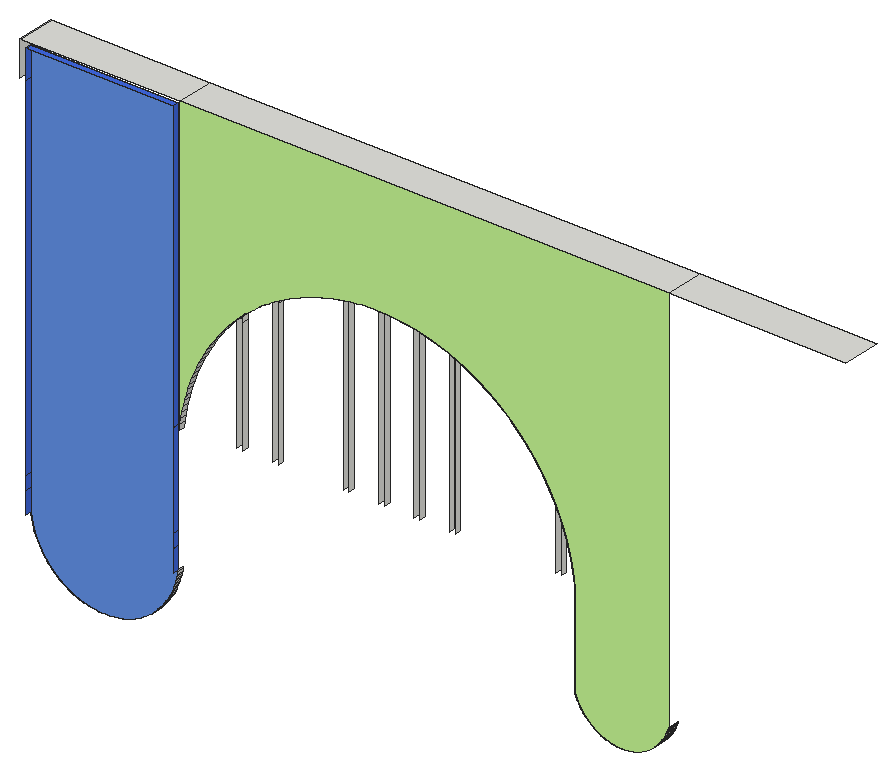
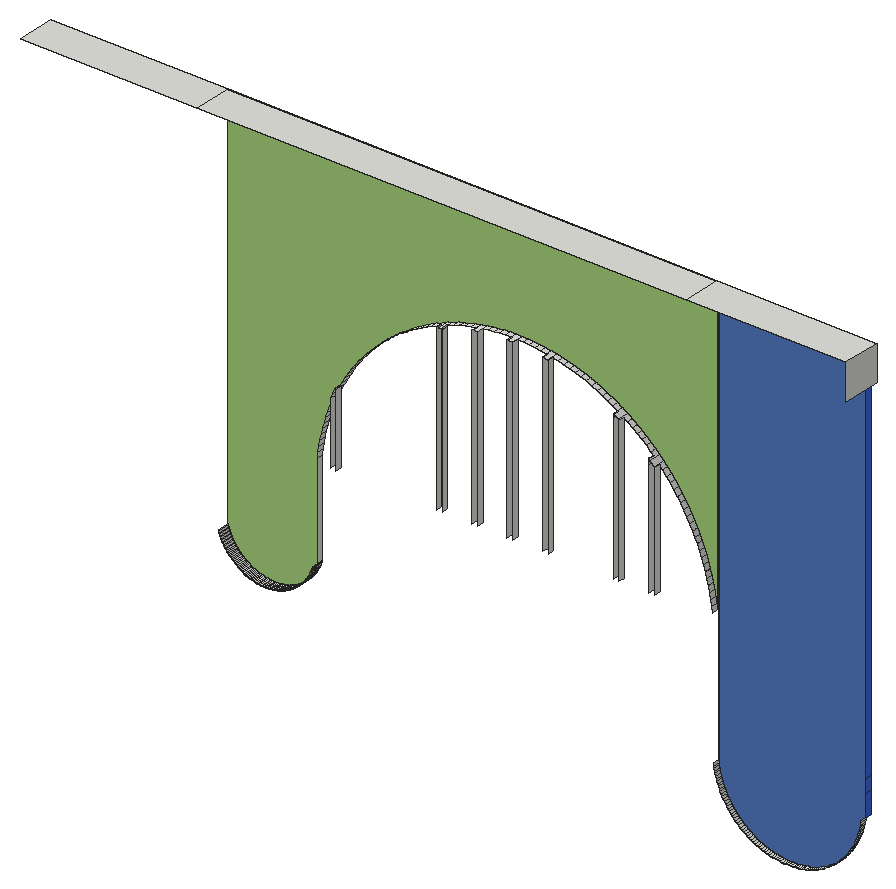
# SketchUp Ruby script. Lengths in inches.
U = 1.inch
M = Sketchup.active_model
def pt(a) = Geom::Point3d.new(a.map { |v| v * U })
def face(e, loops, mat)
  f = e.add_face(loops[0].map { |a| pt(a) })
  loops[1..].each { |l| e.add_face(l.map { |a| pt(a) }).erase! }
  f.material = f.back_material = mat if mat
  f
end
# faces: each face lists its corners as indices into pts; further lists are holes
def faces(e, pts, list, mat = nil) = list.each { |f| face(e, (f[0].is_a?(Array) ? f : [f]).map { |l| l.map { |i| pts[i] } }, mat) }
# xy, xz, yz: faces in a plane at the given z, y or x. An outline is a flat list of corners, or four numbers for a rectangle; further outlines are holes
def ring(l) = l.size == 4 ? [[l[0], l[1]], [l[2], l[1]], [l[2], l[3]], [l[0], l[3]]] : l.each_slice(2).to_a
def flat(e, list, mat, &to3) = list.each { |f| face(e, (f[0].is_a?(Array) ? f : [f]).map { |l| ring(l).map { |u, v| to3.(u, v) } }, mat) }
def xy(e, z, list, mat = nil) = flat(e, list, mat) { |x, y| [x, y, z] }
def xz(e, y, list, mat = nil) = flat(e, list, mat) { |x, z| [x, y, z] }
def yz(e, x, list, mat = nil) = flat(e, list, mat) { |y, z| [x, y, z] }
def lines(e, pts, list) = list.each { |a, b| e.add_line(pt(pts[a]), pt(pts[b])) }
# prism: a flat outline (further loops are holes) pulled along v
def prism(e, loops, v, mat = nil)
  f = face(e, loops, mat); d = Geom::Vector3d.new(v.map { |x| x * U })
  f.pushpull(f.normal.samedirection?(d) ? d.length : -d.length)
end
def box(e, o, s, mat = nil) = prism(e, [[o, [o[0] + s[0], o[1], o[2]], [o[0] + s[0], o[1] + s[1], o[2]], [o[0], o[1] + s[1], o[2]]]], [0, 0, s[2]], mat)
def at(x, y, z, deg = 0) = Geom::Transformation.translation(pt([x, y, z])) * Geom::Transformation.rotation(ORIGIN, Z_AXIS, deg.degrees)
def axes(o, x, y, z) = Geom::Transformation.new([*x, 0, *y, 0, *z, 0, *pt(o).to_a, 1])
def part(name) = M.definitions.add(name)
# library, detail: a bought-in or finely detailed component or shape, given as its bounding box
def library(name, o, s) = part(name).tap { |d| box(d.entities, o, s) }
def detail(e, o, s) = box(e.add_group.entities, o, s)
def put(e, d, t, mat = nil) = e.add_instance(d, t).tap { |i| i.material = mat if mat }
def group(e, t, mat = nil) = e.add_group.tap { |g| g.transformation = t; g.material = mat if mat }.entities
root = M.entities
M.materials.add("[0101_CornflowerBlue]").color = [100, 149, 237]
M.materials.add("[0102_RoyalBlue]").color = [65, 105, 225]
M.materials.add("[Color F02]").color = [204, 255, 153]
xy(root,18.939,[[13.316,5.25,13.684,6.25]])
xy(root,30.001,[[101.892,4.25,102.108,6.25]])
xy(root,81.996,[[60.003,4.25,60.997,6.25]])
xy(root,101,[[1,4.25,26,5.25]],"[0102_RoyalBlue]")
xy(root,102,[[0,4.25,27,10.75],[27,4.25,110,10.75],[110,4.25,140,10.75]])
xz(root,4.25,[[101.892,30.001,102.108,30.001,102.325,30.006,102.541,30.018,102.757,30.034,102.973,30.057,103.1875,30.085,103.402,30.119,103.615,30.158,103.827,30.203,104.037,30.253,104.247,30.309,104.455,30.37,104.661,30.436,104.865,30.508,105.068,30.585,105.268,30.668,105.466,30.755,105.662,30.848,105.856,30.946,106.046,31.048,106.234,31.156,106.419,31.268,106.602,31.386,106.781,31.508,106.957,31.634,107.129,31.765,107.298,31.901,107.463,32.041,107.625,32.185,107.783,32.333,107.937,32.486,108.087,32.642,108.233,32.802,108.375,32.966,108.512,33.134,108.645,33.305,108.774,33.479,108.898,33.657,109.017,33.838,109.131,34.022,109.241,34.209,109.346,34.398,109.446,34.591,109.54,34.785,109.63,34.983,109.715,35.182,109.794,35.384,109.868,35.587,109.937,35.793,110,36,110,102,27,102,27,52,27.124,52.987,27.277,53.969,27.459,54.947,27.669,55.919,27.909,56.885,28.162,57.792,28.176,57.842,28.472,58.792,28.795,59.732,29.147,60.663,29.525,61.582,29.931,62.491,30.363,63.386,30.821,64.269,31.305,65.138,31.815,65.992,32.35,66.83,32.909,67.653,33.492,68.458,34.098,69.246,34.728,70.016,35.38,70.767,36.054,71.499,36.749,72.21,37.465,72.9,38.201,73.569,38.956,74.216,39.731,74.84,40.523,75.441,41.332,76.019,42.159,76.572,43.001,77.101,43.859,77.605,44.73,78.083,45.616,78.536,46.515,78.962,47.426,79.361,48.348,79.733,49.281,80.078,50.223,80.395,51.175,80.684,52.135,80.945,53.102,81.178,54.075,81.382,55.054,81.557,56.038,81.703,57.025,81.82,58.016,81.908,59.009,81.967,60.003,81.996,60.997,81.996,61.991,81.967,62.984,81.908,63.975,81.82,64.962,81.703,65.946,81.557,66.925,81.382,67.898,81.178,68.865,80.945,69.825,80.684,70.777,80.395,71.719,80.078,72.652,79.733,73.574,79.361,74.485,78.962,75.384,78.536,76.27,78.083,77.141,77.605,77.999,77.101,78.841,76.572,79.668,76.019,80.477,75.441,81.269,74.84,82.044,74.216,82.799,73.569,83.535,72.9,84.251,72.21,84.946,71.499,85.62,70.767,86.272,70.016,86.902,69.246,87.508,68.458,88.091,67.653,88.65,66.83,89.185,65.992,89.695,65.138,90.179,64.269,90.637,63.386,91.069,62.491,91.475,61.582,91.853,60.663,92.205,59.732,92.528,58.792,92.824,57.842,93.091,56.885,93.331,55.919,93.541,54.947,93.723,53.969,93.876,52.987,94,52,94,36,94.063,35.793,94.132,35.587,94.206,35.384,94.285,35.182,94.37,34.983,94.46,34.785,94.554,34.591,94.654,34.398,94.759,34.209,94.869,34.022,94.983,33.838,95.102,33.657,95.226,33.479,95.355,33.305,95.488,33.134,95.625,32.966,95.767,32.802,95.913,32.642,96.063,32.486,96.217,32.333,96.375,32.185,96.537,32.041,96.702,31.901,96.871,31.765,97.043,31.634,97.219,31.508,97.398,31.386,97.581,31.268,97.766,31.156,97.954,31.048,98.144,30.946,98.338,30.848,98.534,30.755,98.732,30.668,98.932,30.585,99.135,30.508,99.339,30.436,99.545,30.37,99.753,30.309,99.963,30.253,100.173,30.203,100.385,30.158,100.598,30.119,100.8125,30.085,101.027,30.057,101.243,30.034,101.459,30.018,101.675,30.006]],"[Color F02]")
xz(root,5.25,[[13.316,18.939,13.684,18.939,14.053,18.95,14.421,18.971,14.788,19.004,15.154,19.047,15.519,19.1,15.882,19.165,16.243,19.24,16.601,19.325,16.957,19.421,17.31,19.528,17.66,19.644,18.006,19.771,18.348,19.908,18.686,20.055,19.02,20.212,19.349,20.378,19.673,20.554,19.991,20.739,20.304,20.934,20.611,21.138,20.913,21.35,21.207,21.571,21.496,21.801,21.777,22.039,22.051,22.286,22.318,22.54,22.577,22.802,22.829,23.071,23.073,23.348,23.308,23.632,23.535,23.922,23.753,24.219,23.963,24.522,24.164,24.831,24.355,25.146,24.537,25.467,24.71,25.793,24.873,26.123,25.027,26.458,25.17,26.798,25.304,27.141,25.427,27.489,25.54,27.839,25.643,28.193,25.736,28.55,25.818,28.91,25.889,29.271,25.95,29.635,26,30,26,101,1,101,1,30,1.05,29.635,1.111,29.271,1.182,28.91,1.264,28.55,1.357,28.193,1.46,27.839,1.573,27.489,1.696,27.141,1.83,26.798,1.973,26.458,2.127,26.123,2.29,25.793,2.463,25.467,2.645,25.146,2.836,24.831,3.037,24.522,3.247,24.219,3.465,23.922,3.692,23.632,3.927,23.348,4.171,23.071,4.423,22.802,4.682,22.54,4.949,22.286,5.223,22.039,5.504,21.801,5.793,21.571,6.087,21.35,6.389,21.138,6.696,20.934,7.009,20.739,7.327,20.554,7.651,20.378,7.98,20.212,8.314,20.055,8.652,19.908,8.994,19.771,9.34,19.644,9.69,19.528,10.043,19.421,10.399,19.325,10.757,19.24,11.118,19.165,11.481,19.1,11.846,19.047,12.212,19.004,12.579,18.971,12.947,18.95]],"[0101_CornflowerBlue]")
yz(root,0,[[4.25,96,10.75,102]])
yz(root,1,[[4.25,30,5.25,33.622],[4.25,33.622,5.25,36],[4.25,36,5.25,96],[4.25,96,5.25,101]],"[0102_RoyalBlue]")
yz(root,26,[[4.25,30,5.25,33.622],[4.25,33.622,5.25,36],[4.25,36,5.25,52],[4.25,52,5.25,101]],"[0102_RoyalBlue]")
yz(root,36,[[5.25,52,6.25,71.44]])
yz(root,37,[[5.25,52,6.25,71.44],[5.25,71.44,6.25,72.451]])
yz(root,42,[[5.25,52,6.25,76.466]])
yz(root,43,[[5.25,52,6.25,76.466],[5.25,76.466,6.25,77.101]])
yz(root,54,[[5.25,52,6.25,81.366]])
yz(root,55,[[5.25,52,6.25,81.366],[5.25,81.366,6.25,81.547]])
yz(root,60,[[5.25,52,6.25,81.996]])
yz(root,61,[[5.25,52,6.25,81.996]])
yz(root,66,[[5.25,52,6.25,81.547]])
yz(root,67,[[5.25,52,6.25,81.366]])
yz(root,72,[[5.25,52,6.25,79.733],[5.25,79.733,6.25,79.974]])
yz(root,73,[[5.25,52,6.25,79.593]])
yz(root,90,[[5.25,52,6.25,64.269],[5.25,64.269,6.25,64.59]])
yz(root,91,[[5.25,52,6.25,62.634]])
yz(root,94,[[4.25,36,5.25,52]])
p = [[12.579,6.25,18.971],[12.947,6.25,18.95],[12.947,5.25,18.95],[12.579,5.25,18.971],[13.316,6.25,18.939],[13.316,5.25,18.939],
  [13.684,6.25,18.939],[14.053,6.25,18.95],[14.053,5.25,18.95],[13.684,5.25,18.939],[14.421,6.25,18.971],[14.421,5.25,18.971],
  [11.481,6.25,19.1],[11.846,6.25,19.047],[11.846,5.25,19.047],[11.481,5.25,19.1],[12.212,6.25,19.004],[12.212,5.25,19.004],
  [14.788,6.25,19.004],[14.788,5.25,19.004],[15.154,6.25,19.047],[15.154,5.25,19.047],[15.519,6.25,19.1],[15.519,5.25,19.1],
  [11.118,6.25,19.165],[11.118,5.25,19.165],[15.882,6.25,19.165],[15.882,5.25,19.165],[10.399,6.25,19.325],[10.757,6.25,19.24],
  [10.757,5.25,19.24],[10.399,5.25,19.325],[16.243,6.25,19.24],[16.243,5.25,19.24],[16.601,6.25,19.325],[16.601,5.25,19.325],
  [10.043,6.25,19.421],[10.043,5.25,19.421],[16.957,6.25,19.421],[16.957,5.25,19.421],[9.69,6.25,19.528],[9.69,5.25,19.528],
  [17.31,6.25,19.528],[17.31,5.25,19.528],[9.34,6.25,19.644],[9.34,5.25,19.644],[17.66,6.25,19.644],[17.66,5.25,19.644],
  [8.994,6.25,19.771],[8.994,5.25,19.771],[18.006,6.25,19.771],[18.006,5.25,19.771],[8.652,6.25,19.908],[8.652,5.25,19.908],
  [18.348,6.25,19.908],[18.348,5.25,19.908],[8.314,6.25,20.055],[8.314,5.25,20.055],[18.686,6.25,20.055],[18.686,5.25,20.055],
  [7.98,6.25,20.212],[7.98,5.25,20.212],[19.02,6.25,20.212],[19.02,5.25,20.212],[7.651,6.25,20.378],[7.651,5.25,20.378],
  [19.349,6.25,20.378],[19.349,5.25,20.378],[7.327,6.25,20.554],[7.327,5.25,20.554],[19.673,6.25,20.554],[19.673,5.25,20.554],
  [7.009,6.25,20.739],[7.009,5.25,20.739],[19.991,6.25,20.739],[19.991,5.25,20.739],[6.696,6.25,20.934],[6.696,5.25,20.934],
  [20.304,6.25,20.934],[20.304,5.25,20.934],[6.389,6.25,21.138],[6.389,5.25,21.138],[20.611,6.25,21.138],[20.611,5.25,21.138],
  [6.087,6.25,21.35],[6.087,5.25,21.35],[20.913,6.25,21.35],[20.913,5.25,21.35],[5.793,6.25,21.571],[5.793,5.25,21.571],
  [21.207,6.25,21.571],[21.207,5.25,21.571],[5.504,6.25,21.801],[5.504,5.25,21.801],[21.496,6.25,21.801],[21.496,5.25,21.801],
  [5.223,6.25,22.039],[5.223,5.25,22.039],[21.777,6.25,22.039],[21.777,5.25,22.039],[4.949,6.25,22.286],[4.949,5.25,22.286],
  [22.051,6.25,22.286],[22.051,5.25,22.286],[4.682,6.25,22.54],[4.682,5.25,22.54],[22.318,6.25,22.54],[22.318,5.25,22.54],
  [4.423,6.25,22.802],[4.423,5.25,22.802],[22.577,6.25,22.802],[22.577,5.25,22.802],[4.171,6.25,23.071],[4.171,5.25,23.071],
  [22.829,6.25,23.071],[22.829,5.25,23.071],[3.927,6.25,23.348],[3.927,5.25,23.348],[23.073,6.25,23.348],[23.073,5.25,23.348],
  [3.692,6.25,23.632],[3.692,5.25,23.632],[23.308,6.25,23.632],[23.308,5.25,23.632],[3.465,6.25,23.922],[3.465,5.25,23.922],
  [23.535,6.25,23.922],[23.535,5.25,23.922],[3.247,6.25,24.219],[3.247,5.25,24.219],[23.753,6.25,24.219],[23.753,5.25,24.219],
  [3.037,6.25,24.522],[3.037,5.25,24.522],[23.963,6.25,24.522],[23.963,5.25,24.522],[2.836,6.25,24.831],[2.836,5.25,24.831],
  [24.164,6.25,24.831],[24.164,5.25,24.831],[2.645,6.25,25.146],[2.645,5.25,25.146],[24.355,6.25,25.146],[24.355,5.25,25.146],
  [2.463,6.25,25.467],[2.463,5.25,25.467],[24.537,6.25,25.467],[24.537,5.25,25.467],[2.29,6.25,25.793],[2.29,5.25,25.793],
  [24.71,6.25,25.793],[24.71,5.25,25.793],[2.127,6.25,26.123],[2.127,5.25,26.123],[24.873,6.25,26.123],[24.873,5.25,26.123],
  [1.973,6.25,26.458],[1.973,5.25,26.458],[25.027,6.25,26.458],[25.027,5.25,26.458],[1.83,6.25,26.798],[1.83,5.25,26.798],
  [25.17,6.25,26.798],[25.17,5.25,26.798],[1.696,6.25,27.141],[1.696,5.25,27.141],[25.304,6.25,27.141],[25.304,5.25,27.141],
  [1.573,6.25,27.489],[1.573,5.25,27.489],[25.427,6.25,27.489],[25.427,5.25,27.489],[1.46,6.25,27.839],[1.46,5.25,27.839],
  [25.54,6.25,27.839],[25.54,5.25,27.839],[1.357,6.25,28.193],[1.357,5.25,28.193],[25.643,6.25,28.193],[25.643,5.25,28.193],
  [1.264,6.25,28.55],[1.264,5.25,28.55],[25.736,6.25,28.55],[25.736,5.25,28.55],[1.182,6.25,28.91],[1.182,5.25,28.91],
  [25.818,6.25,28.91],[25.818,5.25,28.91],[1.111,6.25,29.271],[1.111,5.25,29.271],[25.889,6.25,29.271],[25.889,5.25,29.271],
  [1.05,6.25,29.635],[1.05,5.25,29.635],[25.95,6.25,29.635],[25.95,5.25,29.635],[1,6.25,30],[1,5.25,30],
  [26,6.25,30],[26,5.25,30],[101.027,6.25,30.057],[101.243,6.25,30.034],[101.243,4.25,30.034],[101.027,4.25,30.057],
  [101.459,6.25,30.018],[101.459,4.25,30.018],[101.675,6.25,30.006],[101.675,4.25,30.006],[101.892,6.25,30.001],[101.892,4.25,30.001],
  [102.108,6.25,30.001],[102.325,6.25,30.006],[102.325,4.25,30.006],[102.108,4.25,30.001],[102.541,6.25,30.018],[102.541,4.25,30.018],
  [102.757,6.25,30.034],[102.757,4.25,30.034],[102.973,6.25,30.057],[102.973,4.25,30.057],[100.385,6.25,30.158],[100.598,6.25,30.119],
  [100.598,4.25,30.119],[100.385,4.25,30.158],[100.8125,6.25,30.085],[100.8125,4.25,30.085],[103.1875,6.25,30.085],[103.1875,4.25,30.085],
  [103.402,6.25,30.119],[103.402,4.25,30.119],[103.615,6.25,30.158],[103.615,4.25,30.158],[99.963,6.25,30.253],[100.173,6.25,30.203],
  [100.173,4.25,30.203],[99.963,4.25,30.253],[103.827,6.25,30.203],[103.827,4.25,30.203],[104.037,6.25,30.253],[104.037,4.25,30.253],
  [99.545,6.25,30.37],[99.753,6.25,30.309],[99.753,4.25,30.309],[99.545,4.25,30.37],[104.247,6.25,30.309],[104.247,4.25,30.309],
  [104.455,6.25,30.37],[104.455,4.25,30.37],[99.135,6.25,30.508],[99.339,6.25,30.436],[99.339,4.25,30.436],[99.135,4.25,30.508],
  [104.661,6.25,30.436],[104.661,4.25,30.436],[104.865,6.25,30.508],[104.865,4.25,30.508],[98.932,6.25,30.585],[98.932,4.25,30.585],
  [105.068,6.25,30.585],[105.068,4.25,30.585],[98.732,6.25,30.668],[98.732,4.25,30.668],[105.268,6.25,30.668],[105.268,4.25,30.668],
  [98.534,6.25,30.755],[98.534,4.25,30.755],[105.466,6.25,30.755],[105.466,4.25,30.755],[98.144,6.25,30.946],[98.338,6.25,30.848],
  [98.338,4.25,30.848],[98.144,4.25,30.946],[105.662,6.25,30.848],[105.662,4.25,30.848],[105.856,6.25,30.946],[105.856,4.25,30.946],
  [97.954,6.25,31.048],[97.954,4.25,31.048],[106.046,6.25,31.048],[106.046,4.25,31.048],[97.766,6.25,31.156],[97.766,4.25,31.156],
  [106.234,6.25,31.156],[106.234,4.25,31.156],[97.581,6.25,31.268],[97.581,4.25,31.268],[106.419,6.25,31.268],[106.419,4.25,31.268],
  [97.398,6.25,31.386],[97.398,4.25,31.386],[106.602,6.25,31.386],[106.602,4.25,31.386],[97.219,6.25,31.508],[97.219,4.25,31.508],
  [106.781,6.25,31.508],[106.781,4.25,31.508],[97.043,6.25,31.634],[97.043,4.25,31.634],[106.957,6.25,31.634],[106.957,4.25,31.634],
  [96.871,6.25,31.765],[96.871,4.25,31.765],[107.129,6.25,31.765],[107.129,4.25,31.765],[96.702,6.25,31.901],[96.702,4.25,31.901],
  [107.298,6.25,31.901],[107.298,4.25,31.901],[96.537,6.25,32.041],[96.537,4.25,32.041],[107.463,6.25,32.041],[107.463,4.25,32.041],
  [96.375,6.25,32.185],[96.375,4.25,32.185],[107.625,6.25,32.185],[107.625,4.25,32.185],[96.217,6.25,32.333],[96.217,4.25,32.333],
  [107.783,6.25,32.333],[107.783,4.25,32.333],[96.063,6.25,32.486],[96.063,4.25,32.486],[107.937,6.25,32.486],[107.937,4.25,32.486],
  [95.913,6.25,32.642],[95.913,4.25,32.642],[108.087,6.25,32.642],[108.087,4.25,32.642],[95.767,6.25,32.802],[95.767,4.25,32.802],
  [108.233,6.25,32.802],[108.233,4.25,32.802],[95.625,6.25,32.966],[95.625,4.25,32.966],[108.375,6.25,32.966],[108.375,4.25,32.966],
  [95.488,6.25,33.134],[95.488,4.25,33.134],[108.512,6.25,33.134],[108.512,4.25,33.134],[95.355,6.25,33.305],[95.355,4.25,33.305],
  [108.645,6.25,33.305],[108.645,4.25,33.305],[95.226,6.25,33.479],[95.226,4.25,33.479],[108.774,6.25,33.479],[108.774,4.25,33.479],
  [95.102,6.25,33.657],[95.102,4.25,33.657],[108.898,6.25,33.657],[108.898,4.25,33.657],[94.983,6.25,33.838],[94.983,4.25,33.838],
  [109.017,6.25,33.838],[109.017,4.25,33.838],[94.869,6.25,34.022],[94.869,4.25,34.022],[109.131,6.25,34.022],[109.131,4.25,34.022],
  [94.759,6.25,34.209],[94.759,4.25,34.209],[109.241,6.25,34.209],[109.241,4.25,34.209],[94.654,6.25,34.398],[94.654,4.25,34.398],
  [109.346,6.25,34.398],[109.346,4.25,34.398],[94.554,6.25,34.591],[94.554,4.25,34.591],[109.446,6.25,34.591],[109.446,4.25,34.591],
  [94.46,6.25,34.785],[94.46,4.25,34.785],[109.54,6.25,34.785],[109.54,4.25,34.785],[94.37,6.25,34.983],[94.37,4.25,34.983],
  [109.63,6.25,34.983],[109.63,4.25,34.983],[94.285,6.25,35.182],[94.285,4.25,35.182],[109.715,6.25,35.182],[109.715,4.25,35.182],
  [94.206,6.25,35.384],[94.206,4.25,35.384],[109.794,6.25,35.384],[109.794,4.25,35.384],[94.132,6.25,35.587],[94.132,4.25,35.587],
  [109.868,6.25,35.587],[109.868,4.25,35.587],[94.063,6.25,35.793],[94.063,4.25,35.793],[109.937,6.25,35.793],[109.937,4.25,35.793],
  [94,6.25,36],[94,4.25,36],[94,5.25,36],[110,6.25,36],[110,4.25,36],[27,4.25,52],
  [27,5.25,52],[27.124,5.25,52.987],[27.124,4.25,52.987],[93.876,4.25,52.987],[93.876,5.25,52.987],[94,5.25,52],
  [94,4.25,52],[27.277,5.25,53.969],[27.277,4.25,53.969],[93.723,4.25,53.969],[93.723,5.25,53.969],[27.459,5.25,54.947],
  [27.459,4.25,54.947],[93.541,4.25,54.947],[93.541,5.25,54.947],[27.669,5.25,55.919],[27.669,4.25,55.919],[93.331,4.25,55.919],
  [93.331,5.25,55.919],[27.909,5.25,56.885],[27.909,4.25,56.885],[93.091,4.25,56.885],[93.091,5.25,56.885],[28.162,5.25,57.792],
  [28.162,4.25,57.792],[92.824,4.25,57.842],[92.824,5.25,57.842],[28.176,5.25,57.842],[28.176,4.25,57.842],[28.472,5.25,58.792],
  [28.472,4.25,58.792],[92.528,4.25,58.792],[92.528,5.25,58.792],[28.795,5.25,59.732],[28.795,4.25,59.732],[92.205,4.25,59.732],
  [92.205,5.25,59.732],[29.147,5.25,60.663],[29.147,4.25,60.663],[91.853,4.25,60.663],[91.853,5.25,60.663],[29.525,5.25,61.582],
  [29.525,4.25,61.582],[91.475,4.25,61.582],[91.475,5.25,61.582],[29.931,5.25,62.491],[29.931,4.25,62.491],[91.069,4.25,62.491],
  [91.069,5.25,62.491],[30.363,5.25,63.386],[30.363,4.25,63.386],[90.637,6.25,63.386],[91,6.25,62.634],[91,5.25,62.634],
  [90.637,4.25,63.386],[30.821,5.25,64.269],[30.821,4.25,64.269],[90.179,6.25,64.269],[90.179,4.25,64.269],[31.305,5.25,65.138],
  [31.305,4.25,65.138],[89.695,4.25,65.138],[89.695,5.25,65.138],[90,5.25,64.59],[90,6.25,64.59],[31.815,5.25,65.992],
  [31.815,4.25,65.992],[89.185,4.25,65.992],[89.185,5.25,65.992],[32.35,5.25,66.83],[32.35,4.25,66.83],[88.65,4.25,66.83],
  [88.65,5.25,66.83],[32.909,5.25,67.653],[32.909,4.25,67.653],[88.091,4.25,67.653],[88.091,5.25,67.653],[33.492,5.25,68.458],
  [33.492,4.25,68.458],[87.508,4.25,68.458],[87.508,5.25,68.458],[34.098,5.25,69.246],[34.098,4.25,69.246],[86.902,4.25,69.246],
  [86.902,5.25,69.246],[34.728,5.25,70.016],[34.728,4.25,70.016],[86.272,4.25,70.016],[86.272,5.25,70.016],[35.38,5.25,70.767],
  [35.38,4.25,70.767],[85.62,4.25,70.767],[85.62,5.25,70.767],[36,5.25,71.44],[36,6.25,71.44],[36.054,6.25,71.499],
  [36.054,4.25,71.499],[84.946,4.25,71.499],[84.946,5.25,71.499],[36.749,6.25,72.21],[36.749,4.25,72.21],[84.251,4.25,72.21],
  [84.251,5.25,72.21],[37,6.25,72.451],[37,5.25,72.451],[37.465,5.25,72.9],[37.465,4.25,72.9],[83.535,4.25,72.9],
  [83.535,5.25,72.9],[38.201,5.25,73.569],[38.201,4.25,73.569],[82.799,4.25,73.569],[82.799,5.25,73.569],[38.956,5.25,74.216],
  [38.956,4.25,74.216],[82.044,4.25,74.216],[82.044,5.25,74.216],[39.731,5.25,74.84],[39.731,4.25,74.84],[81.269,4.25,74.84],
  [81.269,5.25,74.84],[40.523,5.25,75.441],[40.523,4.25,75.441],[80.477,4.25,75.441],[80.477,5.25,75.441],[41.332,5.25,76.019],
  [41.332,4.25,76.019],[79.668,4.25,76.019],[79.668,5.25,76.019],[42,5.25,76.466],[42,6.25,76.466],[42.159,6.25,76.572],
  [42.159,4.25,76.572],[78.841,4.25,76.572],[78.841,5.25,76.572],[43,6.25,77.101],[43,5.25,77.101],[43.001,5.25,77.101],
  [43.001,4.25,77.101],[77.999,4.25,77.101],[77.999,5.25,77.101],[43.859,5.25,77.605],[43.859,4.25,77.605],[77.141,4.25,77.605],
  [77.141,5.25,77.605],[44.73,5.25,78.083],[44.73,4.25,78.083],[76.27,4.25,78.083],[76.27,5.25,78.083],[45.616,5.25,78.536],
  [45.616,4.25,78.536],[75.384,4.25,78.536],[75.384,5.25,78.536],[46.515,5.25,78.962],[46.515,4.25,78.962],[74.485,4.25,78.962],
  [74.485,5.25,78.962],[47.426,5.25,79.361],[47.426,4.25,79.361],[73.574,4.25,79.361],[73.574,5.25,79.361],[48.348,5.25,79.733],
  [48.348,4.25,79.733],[72.652,6.25,79.733],[73,6.25,79.593],[73,5.25,79.593],[72.652,4.25,79.733],[49.281,5.25,80.078],
  [49.281,4.25,80.078],[71.719,4.25,80.078],[71.719,5.25,80.078],[72,5.25,79.974],[72,6.25,79.974],[50.223,5.25,80.395],
  [50.223,4.25,80.395],[70.777,4.25,80.395],[70.777,5.25,80.395],[51.175,5.25,80.684],[51.175,4.25,80.684],[69.825,4.25,80.684],
  [69.825,5.25,80.684],[52.135,5.25,80.945],[52.135,4.25,80.945],[68.865,4.25,80.945],[68.865,5.25,80.945],[53.102,5.25,81.178],
  [53.102,4.25,81.178],[67.898,4.25,81.178],[67.898,5.25,81.178],[54,5.25,81.366],[54,6.25,81.366],[54.075,6.25,81.382],
  [54.075,4.25,81.382],[66.925,6.25,81.382],[67,6.25,81.366],[67,5.25,81.366],[66.925,4.25,81.382],[55,6.25,81.547],
  [55,5.25,81.547],[55.054,5.25,81.557],[55.054,4.25,81.557],[65.946,4.25,81.557],[65.946,5.25,81.557],[66,5.25,81.547],
  [66,6.25,81.547],[56.038,5.25,81.703],[56.038,4.25,81.703],[64.962,4.25,81.703],[64.962,5.25,81.703],[57.025,5.25,81.82],
  [57.025,4.25,81.82],[63.975,4.25,81.82],[63.975,5.25,81.82],[58.016,5.25,81.908],[58.016,4.25,81.908],[62.984,4.25,81.908],
  [62.984,5.25,81.908],[59.009,5.25,81.967],[59.009,4.25,81.967],[61.991,4.25,81.967],[61.991,5.25,81.967],[60,5.25,81.996],
  [60,6.25,81.996],[60.003,6.25,81.996],[60.003,4.25,81.996],[60.997,6.25,81.996],[61,6.25,81.996],[61,5.25,81.996],
  [60.997,4.25,81.996],[36,6.25,71.5625],[42,6.25,76.572],[54,6.25,81.557],[66,6.25,81.557],[91,6.25,64.269],
  [91,6.25,64.59],[73,6.25,79.733],[73,6.25,79.974],[67,6.25,81.547],[37,6.25,72.555]]
faces(root,p,[[0,1,2,3],[1,4,5,2],[6,7,8,9],[7,10,11,8],[12,13,14,15],[13,16,17,14],[16,0,3,17],[10,18,19,11],
  [18,20,21,19],[20,22,23,21],[24,12,15,25],[22,26,27,23],[28,29,30,31],[29,24,25,30],[26,32,33,27],[32,34,35,33],
  [36,28,31,37],[34,38,39,35],[40,36,37,41],[38,42,43,39],[44,40,41,45],[42,46,47,43],[48,44,45,49],[46,50,51,47],
  [52,48,49,53],[50,54,55,51],[56,52,53,57],[54,58,59,55],[60,56,57,61],[58,62,63,59],[64,60,61,65],[62,66,67,63],
  [68,64,65,69],[66,70,71,67],[72,68,69,73],[70,74,75,71],[76,72,73,77],[74,78,79,75],[80,76,77,81],[78,82,83,79],
  [84,80,81,85],[82,86,87,83],[88,84,85,89],[86,90,91,87],[92,88,89,93],[90,94,95,91],[96,92,93,97],[94,98,99,95],
  [100,96,97,101],[98,102,103,99],[104,100,101,105],[102,106,107,103],[108,104,105,109],[106,110,111,107],[112,108,109,113],[110,114,115,111],
  [116,112,113,117],[114,118,119,115],[120,116,117,121],[118,122,123,119],[124,120,121,125],[122,126,127,123],[128,124,125,129],[126,130,131,127],
  [132,128,129,133],[130,134,135,131],[136,132,133,137],[134,138,139,135],[140,136,137,141],[138,142,143,139],[144,140,141,145],[142,146,147,143],
  [148,144,145,149],[146,150,151,147],[152,148,149,153],[150,154,155,151],[156,152,153,157],[154,158,159,155],[160,156,157,161],[158,162,163,159],
  [164,160,161,165],[162,166,167,163],[168,164,165,169],[166,170,171,167],[172,168,169,173],[170,174,175,171],[176,172,173,177],[174,178,179,175],
  [180,176,177,181],[178,182,183,179],[184,180,181,185],[182,186,187,183],[188,184,185,189],[186,190,191,187],[192,188,189,193],[190,194,195,191],
  [196,192,193,197],[194,198,199,195],[200,201,202,203],[201,204,205,202],[204,206,207,205],[206,208,209,207],[210,211,212,213],[211,214,215,212],
  [214,216,217,215],[216,218,219,217],[220,221,222,223],[221,224,225,222],[224,200,203,225],[218,226,227,219],[226,228,229,227],[228,230,231,229],
  [232,233,234,235],[233,220,223,234],[230,236,237,231],[236,238,239,237],[240,241,242,243],[241,232,235,242],[238,244,245,239],[244,246,247,245],
  [248,249,250,251],[249,240,243,250],[246,252,253,247],[252,254,255,253],[256,248,251,257],[254,258,259,255],[260,256,257,261],[258,262,263,259],
  [264,260,261,265],[262,266,267,263],[268,269,270,271],[269,264,265,270],[266,272,273,267],[272,274,275,273],[276,268,271,277],[274,278,279,275],
  [280,276,277,281],[278,282,283,279],[284,280,281,285],[282,286,287,283],[288,284,285,289],[286,290,291,287],[292,288,289,293],[290,294,295,291],
  [296,292,293,297],[294,298,299,295],[300,296,297,301],[298,302,303,299],[304,300,301,305],[302,306,307,303],[308,304,305,309],[306,310,311,307],
  [312,308,309,313],[310,314,315,311],[316,312,313,317],[314,318,319,315],[320,316,317,321],[318,322,323,319],[324,320,321,325],[322,326,327,323],
  [328,324,325,329],[326,330,331,327],[332,328,329,333],[330,334,335,331],[336,332,333,337],[334,338,339,335],[340,336,337,341],[338,342,343,339],
  [344,340,341,345],[342,346,347,343],[348,344,345,349],[346,350,351,347],[352,348,349,353],[350,354,355,351],[356,352,353,357],[354,358,359,355],
  [360,356,357,361],[358,362,363,359],[364,360,361,365],[362,366,367,363],[368,364,365,369],[366,370,371,367],[372,368,369,373],[370,374,375,371],
  [376,372,373,377],[374,378,379,375],[380,376,377,381],[378,382,383,379],[384,380,381,385],[382,386,387,383],[388,384,385,389],[386,390,391,387],
  [392,388,389,393],[390,394,395,391],[396,392,393,397,398],[394,399,400,395],[401,402,403,404],[405,406,407,408],[404,403,409,410],[411,412,406,405],
  [410,409,413,414],[415,416,412,411],[414,413,417,418],[419,420,416,415],[418,417,421,422],[423,424,420,419],[422,421,425,426],[427,428,424,423],
  [426,425,429,430],[430,429,431,432],[433,434,428,427],[432,431,435,436],[437,438,434,433],[436,435,439,440],[441,442,438,437],[440,439,443,444],
  [445,446,442,441],[444,443,447,448],[449,450,446,445],[448,447,451,452],[453,454,455,450,449,456],[452,451,457,458],[459,453,456,460],[458,457,461,462],
  [463,464,465,466,459,460],[462,461,467,468],[469,470,464,463],[468,467,471,472],[473,474,470,469],[472,471,475,476],[477,478,474,473],[476,475,479,480],
  [481,482,478,477],[480,479,483,484],[485,486,482,481],[484,483,487,488],[489,490,486,485],[488,487,491,492],[493,494,490,489],[492,491,495,496,497,498],
  [499,500,494,493],[497,501,502,498],[503,504,500,499],[501,505,506,507,508,502],[509,510,504,503],[508,507,511,512],[513,514,510,509],[512,511,515,516],
  [517,518,514,513],[516,515,519,520],[521,522,518,517],[520,519,523,524],[525,526,522,521],[524,523,527,528],[529,530,526,525],[528,527,531,532,533,534],
  [535,536,530,529],[533,537,538,539,540,534],[541,542,536,535],[540,539,543,544],[545,546,542,541],[544,543,547,548],[549,550,546,545],[548,547,551,552],
  [553,554,550,549],[552,551,555,556],[557,558,554,553],[556,555,559,560],[561,562,558,557],[560,559,563,564],[565,566,567,562,561,568],[564,563,569,570],
  [571,572,573,574,565,568],[570,569,575,576],[577,578,572,571],[576,575,579,580],[581,582,578,577],[580,579,583,584],[585,586,582,581],[584,583,587,588],
  [589,590,586,585],[588,587,591,592,593,594],[595,596,597,590,589,598],[593,599,600,601,602,594],[603,604,605,606,595,598],[602,601,607,608],[609,610,604,603],[608,607,611,612],
  [613,614,610,609],[612,611,615,616],[617,618,614,613],[616,615,619,620],[621,622,618,617],[620,619,623,624,625,626],[627,628,629,622,621,630]])
lines(root,p,[[496,631],[532,632],[592,633],[606,634],[635,636],[637,638],[454,635],[566,637],[596,639],[505,640]])
